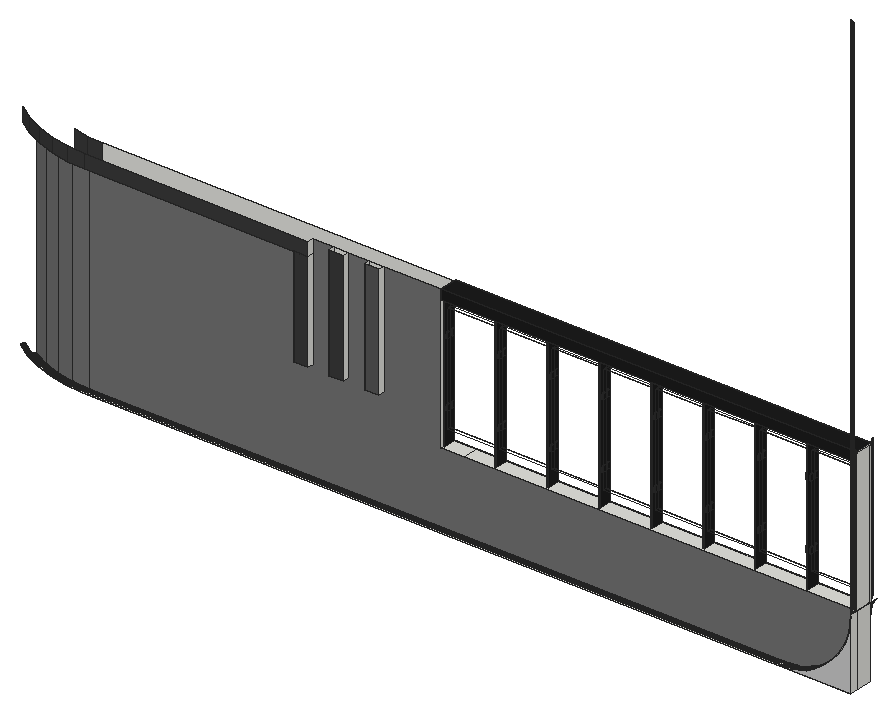
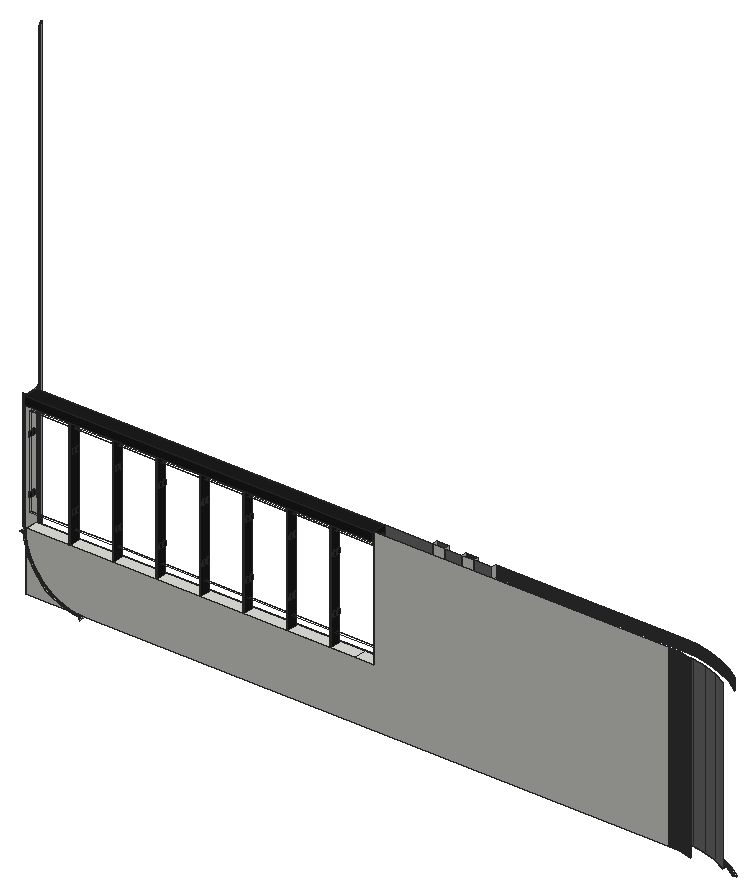
# SketchUp Ruby script. Lengths in inches.
U = 1.inch
M = Sketchup.active_model
def pt(a) = Geom::Point3d.new(a.map { |v| v * U })
def face(e, loops, mat)
  f = e.add_face(loops[0].map { |a| pt(a) })
  loops[1..].each { |l| e.add_face(l.map { |a| pt(a) }).erase! }
  f.material = f.back_material = mat if mat
  f
end
# faces: each face lists its corners as indices into pts; further lists are holes
def faces(e, pts, list, mat = nil) = list.each { |f| face(e, (f[0].is_a?(Array) ? f : [f]).map { |l| l.map { |i| pts[i] } }, mat) }
# xy, xz, yz: faces in a plane at the given z, y or x. An outline is a flat list of corners, or four numbers for a rectangle; further outlines are holes
def ring(l) = l.size == 4 ? [[l[0], l[1]], [l[2], l[1]], [l[2], l[3]], [l[0], l[3]]] : l.each_slice(2).to_a
def flat(e, list, mat, &to3) = list.each { |f| face(e, (f[0].is_a?(Array) ? f : [f]).map { |l| ring(l).map { |u, v| to3.(u, v) } }, mat) }
def xy(e, z, list, mat = nil) = flat(e, list, mat) { |x, y| [x, y, z] }
def xz(e, y, list, mat = nil) = flat(e, list, mat) { |x, z| [x, y, z] }
def yz(e, x, list, mat = nil) = flat(e, list, mat) { |y, z| [x, y, z] }
def lines(e, pts, list) = list.each { |a, b| e.add_line(pt(pts[a]), pt(pts[b])) }
# prism: a flat outline (further loops are holes) pulled along v
def prism(e, loops, v, mat = nil)
  f = face(e, loops, mat); d = Geom::Vector3d.new(v.map { |x| x * U })
  f.pushpull(f.normal.samedirection?(d) ? d.length : -d.length)
end
def box(e, o, s, mat = nil) = prism(e, [[o, [o[0] + s[0], o[1], o[2]], [o[0] + s[0], o[1] + s[1], o[2]], [o[0], o[1] + s[1], o[2]]]], [0, 0, s[2]], mat)
def at(x, y, z, deg = 0) = Geom::Transformation.translation(pt([x, y, z])) * Geom::Transformation.rotation(ORIGIN, Z_AXIS, deg.degrees)
def axes(o, x, y, z) = Geom::Transformation.new([*x, 0, *y, 0, *z, 0, *pt(o).to_a, 1])
def part(name) = M.definitions.add(name)
# library, detail: a bought-in or finely detailed component or shape, given as its bounding box
def library(name, o, s) = part(name).tap { |d| box(d.entities, o, s) }
def detail(e, o, s) = box(e.add_group.entities, o, s)
def put(e, d, t, mat = nil) = e.add_instance(d, t).tap { |i| i.material = mat if mat }
def group(e, t, mat = nil) = e.add_group.tap { |g| g.transformation = t; g.material = mat if mat }.entities
root = M.entities
M.materials.add("[0131_Silver]").color = [28, 28, 28]
M.materials.add("[Cladding Stucco White]").color = [200, 200, 200]
M.materials.add("[Color M05]").color = [114, 114, 114]
M.materials.add("[Color M06]").color = [86, 86, 86]
M.materials.add("[Color M07]").color = [58, 58, 58]
M.materials.add("[Translucent_Glass_Blue]").color = [255, 255, 255]
M.materials["[Translucent_Glass_Blue]"].alpha = 0
c1 = part("Group\#11")
xy(c1.entities,0,[[0,0,0.39,2.125]],"[0131_Silver]")
xy(c1.entities,1.5,[[0,0,0.39,2.125]],"[0131_Silver]")
xz(c1.entities,0,[[0,0,0.39,1.5]],"[0131_Silver]")
xz(c1.entities,2.125,[[0,0,0.39,1.5]],"[0131_Silver]")
yz(c1.entities,0,[[0,0,2.125,1.5]],"[0131_Silver]")
yz(c1.entities,0.39,[[0,0,2.125,1.5]],"[0131_Silver]")
c2 = part("Glass railing panel")
xy(c2.entities,0,[[-0.59,0,0,63.98]])
xy(c2.entities,37.71,[[-0.59,0,0,63.98]])
xz(c2.entities,0,[[-0.59,0,0,37.71]])
xz(c2.entities,63.98,[[-0.59,0,0,37.71]])
yz(c2.entities,-0.59,[[0,0,63.98,37.71]])
yz(c2.entities,0,[[0,0,63.98,0,63.98,37.71,0,37.71,0,30.53,1.75,30.53,1.75,28.71,0,28.71],[-0.4,28.71,0,30.53],[0,28.71,1.75,30.53]])
p = [[0,63.98,30.53],[0.39,63.98,30.53]]
lines(c2.entities,p,[[0,1]])
put(c2.entities,c1,axes([0,62.22,28.71],[1,0,0],[0,1.01246,0],[0,0,1.2158]))
put(c2.entities,c1,axes([0,62.22,6.27],[1,0,0],[0,1.01246,0],[0,0,1.2158]))
put(c2.entities,c1,axes([0,0.6,28.71],[1,0,0],[0,1.01246,0],[0,0,1.2158]))
put(c2.entities,c1,axes([0,0.6,6.27],[1,0,0],[0,1.01246,0],[0,0,1.2158]))
put(c2.entities,c1,axes([-0.98,0.6,28.71],[1,0,0],[0,1.01246,0],[0,0,1.2158]))
put(c2.entities,c1,axes([-0.98,62.22,6.27],[1,0,0],[0,1.01246,0],[0,0,1.2158]))
put(c2.entities,c1,axes([-0.98,0.6,6.27],[1,0,0],[0,1.01246,0],[0,0,1.2158]))
put(c2.entities,c1,axes([-0.98,62.22,28.71],[1,0,0],[0,1.01246,0],[0,0,1.2158]))
c3 = part("Group\#1")
xz(c3.entities,0,[[0,0,1.97,38.58]])
xz(c3.entities,1.97,[[0,0,1.97,38.58]])
yz(c3.entities,0,[[0,0,1.97,37.71]])
yz(c3.entities,1.97,[[0,0,1.97,37.71]])
c4 = part("Glass railing section")
xy(c4.entities,37.71,[[2.51,0,3.15,0.39,3.15,0]])
xy(c4.entities,37.71,[[0,0,0.54,520.67],[2.51,0,2.51,63.58,3.15,0.39],[3.15,0.39,2.51,63.58,2.51,520.67,3.15,520.67]],"[0131_Silver]")
xy(c4.entities,38.58,[[0.54,496.0625,2.51,520.67]])
xy(c4.entities,38.58,[[0.54,0,2.51,496.0625]],"[0131_Silver]")
xy(c4.entities,40.46,[[0,0,3.15,520.67]],"[0131_Silver]")
xz(c4.entities,0,[[0,37.71,0.54,37.71,0.54,38.58,2.51,38.58,2.51,37.71,3.15,37.71,3.15,40.46,0,40.46]],"[0131_Silver]")
xz(c4.entities,520.67,[[0,37.71,0,40.46,3.15,40.46,3.15,37.71,2.51,37.71,2.51,38.58,0.54,38.58,0.54,37.71]])
yz(c4.entities,0,[[0,37.71,520.67,40.46]],"[0131_Silver]")
yz(c4.entities,0.54,[[496.0625,37.71,520.67,38.58]])
yz(c4.entities,0.54,[[0,37.71,496.0625,38.58]],"[0131_Silver]")
yz(c4.entities,2.51,[[0,37.71,496.0625,38.58],[496.0625,37.71,520.67,38.58]])
yz(c4.entities,3.15,[[0,37.71,520.67,40.46]],"[0131_Silver]")
put(c4.entities,c2,axes([1.8,65.35,3.9375],[1,0,0],[0,0.98769,0],[0,0,0.8225]),"[Translucent_Glass_Blue]")
put(c4.entities,c2,axes([1.8,130.31,3.9375],[1,0,0],[0,0.98769,0],[0,0,0.8225]),"[Translucent_Glass_Blue]")
put(c4.entities,c2,axes([1.8,195.28,3.9375],[1,0,0],[0,0.98769,0],[0,0,0.8225]),"[Translucent_Glass_Blue]")
put(c4.entities,c2,axes([1.8,260.24,3.9375],[1,0,0],[0,0.98769,0],[0,0,0.8225]),"[Translucent_Glass_Blue]")
put(c4.entities,c2,axes([1.8,325.2,3.9375],[1,0,0],[0,0.98769,0],[0,0,0.8225]),"[Translucent_Glass_Blue]")
put(c4.entities,c2,axes([1.8,390.16,3.9375],[1,0,0],[0,0.98769,0],[0,0,0.8225]),"[Translucent_Glass_Blue]")
put(c4.entities,c2,axes([1.8,455.12,3.9375],[1,0,0],[0,0.98769,0],[0,0,0.8225]),"[Translucent_Glass_Blue]")
put(c4.entities,c2,axes([1.8,0.39,3.9375],[1,0,0],[0,0.98769,0],[0,0,0.8225]),"[Translucent_Glass_Blue]")
put(c4.entities,c3,at(0.54,128.9375,0),"[0131_Silver]")
g1 = group(c4.entities,at(0.54,63.98,0),"[0131_Silver]")
xz(g1,0,[[0,0,1.97,38.58]])
xz(g1,1.97,[[0,0,1.97,38.58]])
yz(g1,0,[[0,0,1.97,37.71]])
yz(g1,1.97,[[0,0,1.97,37.71]])
put(c4.entities,c3,at(0.54,193.9,0),"[0131_Silver]")
put(c4.entities,c3,at(0.54,258.86,0),"[0131_Silver]")
put(c4.entities,c3,at(0.54,323.82,0),"[0131_Silver]")
put(c4.entities,c3,at(0.54,388.78,0),"[0131_Silver]")
put(c4.entities,c3,at(0.54,453.74,0),"[0131_Silver]")
put(c4.entities,c3,at(0.54,518.7,0),"[0131_Silver]")
c5 = part("Glass+Railing")
put(c5.entities,c4,axes([0,0,0],[1,0,0],[0,0.95652,0],[0,0,1]),"[0131_Silver]")
xy(root,126,[[142.019,1,154.019,2.33],[142.019,2.33,154.019,5.061]])
xy(root,126.103,[[24.213,1.209,24.213,1.212,21.145,1.413,21.144,1.41],[24.213,1.209,24.257,1.209,24.213,1.212],[21.144,1.41,21.145,1.413,18.093,2.02,18.092,2.017],[18.092,2.017,18.093,2.02,15.146,3.02,15.145,3.018],[21.264,2.317,21.264,2.32,18.329,2.903,18.328,2.901],
  [18.328,2.901,18.329,2.903,15.496,3.865,15.495,3.863],[15.145,3.018,15.146,3.02,12.355,4.397,12.353,4.394],[15.495,3.863,15.496,3.865,12.812,5.189,12.811,5.186],[12.353,4.394,12.355,4.397,9.767,6.126,9.765,6.123]])
xy(root,126.14,[[24.217,1.32,24.217,1.322,21.159,1.523,21.159,1.52],[24.217,1.32,24.26,1.32,24.217,1.322],[21.159,1.52,21.159,1.523,18.121,2.127,18.121,2.124],[18.121,2.124,18.121,2.127,15.188,3.123,15.187,3.12],[21.249,2.207,21.25,2.21,18.301,2.796,18.3,2.793],
  [18.3,2.793,18.301,2.796,15.453,3.763,15.452,3.76],[15.187,3.12,15.188,3.123,12.41,4.493,12.409,4.49],[15.452,3.76,15.453,3.763,12.756,5.093,12.755,5.09],[12.409,4.49,12.41,4.493,9.835,6.214,9.833,6.211]])
xy(root,126.166,[[24.221,1.433,24.221,1.436,21.174,1.636,21.174,1.633],[24.221,1.433,24.264,1.433,24.221,1.436],[21.174,1.633,21.174,1.636,18.151,2.237,18.15,2.234],[24.236,1.897,24.236,1.9,21.235,2.097,21.234,2.094],[24.236,1.897,24.279,1.897,24.236,1.9],
  [21.234,2.094,21.235,2.097,18.271,2.686,18.27,2.684],[18.15,2.234,18.151,2.237,15.232,3.228,15.231,3.225],[18.27,2.684,18.271,2.686,15.41,3.658,15.409,3.655],[15.231,3.225,15.232,3.228,12.467,4.591,12.466,4.589],[15.409,3.655,15.41,3.658,12.7,4.994,12.698,4.992],
  [12.466,4.589,12.467,4.591,9.904,6.304,9.902,6.302]])
xy(root,126.182,[[24.224,1.549,24.225,1.552,21.189,1.751,21.189,1.748],[24.224,1.549,24.268,1.549,24.225,1.552],[21.189,1.748,21.189,1.751,18.181,2.349,18.18,2.346],[24.232,1.782,24.232,1.785,21.22,1.982,21.219,1.979],[24.232,1.782,24.276,1.782,24.232,1.785],
  [21.219,1.979,21.22,1.982,18.241,2.574,18.24,2.572],[18.18,2.346,18.181,2.349,15.276,3.335,15.275,3.332],[18.24,2.572,18.241,2.574,15.365,3.551,15.364,3.548],[15.275,3.332,15.276,3.335,12.525,4.692,12.524,4.689],[15.364,3.548,15.365,3.551,12.642,4.894,12.64,4.891],
  [12.524,4.689,12.525,4.692,9.974,6.396,9.973,6.394]])
xy(root,126.1875,[[24.228,1.665,24.228,1.668,21.204,1.866,21.204,1.863],[24.228,1.665,24.272,1.665,24.228,1.668],[21.204,1.863,21.204,1.866,18.211,2.462,18.211,2.46,18.21,2.459],[18.21,2.459,18.211,2.46,18.211,2.462,15.321,3.443,15.32,3.441,15.32,3.44],[15.32,3.44,15.32,3.441,15.321,3.443,12.583,4.793,12.583,4.791,12.582,4.79],
  [12.582,4.79,12.583,4.791,12.583,4.793,10.046,6.488,10.044,6.486]])
xy(root,137.896,[[83.599,2.33,87.474,5.061],[87.474,2.33,153.974,5.061]])
xy(root,142.9375,[[59.529,1.33,61.967,2.33],[65.529,1.33,67.967,2.33],[71.529,1.33,73.967,2.33]])
xz(root,1,[[142.019,126,154.019,126,154.019,138,153.916,136.434,153.61,134.894,153.105,133.408,152.411,132,151.539,130.695,150.504,129.515,149.324,128.48,148.019,127.608,146.611,126.913,145.124,126.409,143.585,126.103]],"[Cladding Stucco White]")
xz(root,1.33,[[71.529,142.9375,73.967,162]],"[Color M06]")
xz(root,1.33,[[59.529,142.9375,61.967,159.6875],[65.529,142.9375,67.967,162],[24.217,159.6875,61.967,162]],"[Color M07]")
xz(root,2.33,[[65.529,142.9375,67.967,162],[71.529,142.9375,73.967,162]])
xz(root,2.33,[[24.25,126,154.019,126,154.019,162,153.974,137.896,83.599,137.896,83.599,162,73.967,162,73.967,142.9375,71.529,142.9375,71.529,162,67.967,162,67.967,142.9375,65.529,142.9375,65.529,162,61.967,162,61.967,142.9375,59.529,142.9375,59.529,159.6875,24.25,159.6875]],"[Color M05]")
xz(root,5.061,[[24.25,126,24.25,162,83.599,162,83.599,137.896,153.974,137.896,154.019,162,154.019,126]])
yz(root,59.529,[[1.33,142.9375,2.33,159.6875]])
yz(root,61.967,[[1.33,142.9375,2.33,159.6875],[1.33,159.6875,2.33,162]])
yz(root,65.529,[[1.33,142.9375,2.33,162]])
yz(root,67.967,[[1.33,142.9375,2.33,162]])
yz(root,71.529,[[1.33,142.9375,2.33,162]])
yz(root,73.967,[[1.33,142.9375,2.33,162]])
yz(root,83.599,[[2.33,137.896,5.061,162]])
yz(root,154.019,[[1,126,2.33,138],[2.33,126,5.061,138],[2.33,138,5.061,162]])
p = [[24.25,1,126],[24.253,1.102,126.056],[21.131,1.307,126.056],[21.117,1.205,126],[24.207,1.003,126],[21.13,1.304,126.056],
  [21.117,1.202,126],[24.206,1,126],[24.21,1.102,126.056],[140.688,1,126],[142.019,1,126],[141.916,1.102,126.056],
  [140.79,1.102,126.056],[142.019,2.33,126],[141.916,2.228,126.056],[142.123,1.107,126.045],[143.585,1,126.103],[143.58,1.107,126.14],
  [142.123,2.33,126.045],[142.123,5.061,126.045],[142.123,6.284,126.045],[142.019,6.391,126],[142.019,5.061,126],[142.23,1.216,126.083],
  [143.576,1.216,126.171],[142.23,2.33,126.083],[142.23,5.061,126.083],[142.23,6.175,126.083],[18.064,1.914,126.056],[18.038,1.815,126],
  [18.065,1.917,126.056],[18.038,1.818,126],[15.104,2.919,126.056],[15.065,2.824,126],[15.105,2.921,126.056],[15.066,2.827,126],
  [21.291,2.524,126],[21.278,2.423,126.056],[24.247,2.228,126.056],[24.25,2.33,126],[24.29,2.228,126.056],[24.294,2.33,126],
  [21.291,2.527,126],[21.291,2.524,126.002],[21.278,2.426,126.056],[140.688,2.33,126],[140.79,2.228,126.056],[24.25,2.33,159.6875],
  [21.291,2.524,159.6875],[18.383,3.103,126],[18.356,3.004,126.056],[18.383,3.106,126],[18.383,3.103,126.002],[18.357,3.007,126.056],
  [18.383,3.103,159.6875],[12.3,4.302,126.056],[12.249,4.213,126],[12.301,4.304,126.056],[12.25,4.215,126],[15.575,4.056,126],
  [15.536,3.961,126.056],[15.576,4.059,126],[15.575,4.056,126.002],[15.537,3.964,126.056],[15.575,4.056,159.6875],[12.915,5.368,126],
  [12.864,5.279,126.056],[12.917,5.37,126],[12.915,5.368,126.002],[12.865,5.281,126.056],[12.915,5.368,159.6875],[9.7,6.038,126.056],
  [9.638,5.957,126],[9.702,6.041,126.056],[9.64,5.96,126],[24.25,5.061,126],[21.647,5.231,126],[21.647,5.231,162],
  [24.25,5.061,162],[19.089,5.74,126],[19.089,5.74,162],[145.124,1,126.409],[145.115,1.107,126.445],[24.257,1.209,126.103],
  [24.213,1.212,126.103],[21.145,1.413,126.103],[21.144,1.41,126.103],[24.213,1.209,126.103],[141.81,1.209,126.103],[140.897,1.209,126.103],
  [141.81,2.121,126.103],[145.106,1.216,126.476],[24.26,1.32,126.14],[24.217,1.322,126.14],[21.159,1.523,126.14],[21.159,1.52,126.14],
  [24.217,1.32,126.14],[141.699,1.32,126.14],[141.008,1.32,126.14],[141.699,2.011,126.14],[142.339,1.327,126.114],[143.573,1.327,126.195],
  [142.339,6.064,126.114],[142.339,2.33,126.114],[142.339,5.061,126.114],[18.092,2.017,126.103],[18.093,2.02,126.103],[24.264,1.433,126.166],
  [24.221,1.436,126.166],[21.174,1.636,126.166],[21.174,1.633,126.166],[24.221,1.433,126.166],[141.585,1.433,126.166],[141.121,1.433,126.166],
  [141.585,1.897,126.166],[142.449,1.439,126.139],[143.57,1.439,126.213],[142.449,5.952,126.139],[142.449,2.33,126.139],[142.449,5.061,126.139],
  [18.121,2.124,126.14],[142.561,1.552,126.157],[143.569,1.552,126.223],[142.561,2.33,126.157],[142.561,5.061,126.157],[142.561,5.839,126.157],
  [18.15,2.234,126.166],[18.121,2.127,126.14],[15.145,3.018,126.103],[15.146,3.02,126.103],[24.279,1.897,126.166],[24.283,2.011,126.14],
  [24.24,2.013,126.139],[21.25,2.21,126.14],[21.249,2.207,126.14],[21.235,2.097,126.166],[24.236,1.9,126.166],[24.24,2.011,126.14],
  [141.121,1.897,126.166],[141.008,2.011,126.14],[15.187,3.12,126.14],[24.287,2.121,126.103],[21.264,2.32,126.103],[21.264,2.317,126.103],
  [24.243,2.121,126.103],[140.897,2.121,126.103],[143.126,2.114,126.142],[143.014,2.004,126.159],[143.573,2.004,126.195],[143.576,2.114,126.171],
  [143.126,5.277,126.142],[143.014,5.388,126.159],[143.014,5.061,126.159],[143.014,2.33,126.159],[143.126,2.33,126.142],[143.126,5.061,126.142],
  [15.231,3.225,126.166],[15.188,3.123,126.14],[18.3,2.793,126.14],[18.271,2.686,126.166],[143.237,2.223,126.118],[143.58,2.223,126.14],
  [143.237,5.168,126.118],[143.237,2.33,126.118],[143.237,5.061,126.118],[145.106,2.114,126.476],[145.115,2.223,126.445],[18.328,2.901,126.103],
  [18.301,2.796,126.14],[143.346,2.33,126.087],[143.585,2.33,126.103],[143.346,5.061,126.087],[145.124,2.33,126.409],[18.329,2.903,126.103],
  [143.585,5.061,126.103],[145.124,5.061,126.409],[15.452,3.76,126.14],[15.41,3.658,126.166],[15.495,3.863,126.103],[15.453,3.763,126.14],
  [12.353,4.394,126.103],[12.355,4.397,126.103],[15.496,3.865,126.103],[12.409,4.49,126.14],[12.466,4.589,126.166],[12.41,4.493,126.14],
  [12.755,5.09,126.14],[12.7,4.994,126.166],[12.811,5.186,126.103],[12.756,5.093,126.14],[12.812,5.189,126.103],[9.765,6.123,126.103],
  [9.767,6.126,126.103],[9.833,6.211,126.14],[9.902,6.302,126.166],[9.835,6.214,126.14],[143.58,5.168,126.14],[145.115,5.168,126.445],
  [143.576,5.277,126.171],[145.106,5.277,126.476],[143.573,5.388,126.195],[145.1,1.327,126.499],[145.096,1.439,126.516],[24.268,1.549,126.182],
  [24.225,1.552,126.182],[21.189,1.751,126.182],[21.189,1.748,126.182],[24.224,1.549,126.182],[141.47,1.549,126.182],[141.237,1.549,126.182],
  [141.47,1.782,126.182],[145.093,1.552,126.526],[24.272,1.665,126.1875],[24.228,1.668,126.1875],[21.204,1.866,126.1875],[21.204,1.865,126.1875],
  [21.204,1.863,126.1875],[24.228,1.665,126.1875],[141.353,1.665,126.1875],[18.18,2.346,126.182],[18.151,2.237,126.166],[142.674,1.665,126.168],
  [143.569,1.665,126.227],[142.674,2.33,126.168],[142.674,5.061,126.168],[142.674,5.726,126.168],[145.092,1.665,126.53],[21.22,1.982,126.182],
  [21.219,1.979,126.182],[24.232,1.782,126.182],[24.276,1.782,126.182],[24.232,1.785,126.182],[141.237,1.782,126.182],[142.788,1.779,126.172],
  [143.569,1.779,126.223],[142.788,2.33,126.172],[142.788,5.061,126.172],[142.788,5.613,126.172],[145.093,1.779,126.526],[18.21,2.459,126.1875],
  [18.181,2.349,126.182],[21.234,2.094,126.166],[24.236,1.897,126.166],[142.901,1.892,126.169],[143.57,1.892,126.213],[142.901,2.33,126.169],
  [142.901,5.061,126.169],[142.901,5.5,126.169],[145.096,1.892,126.516],[18.24,2.572,126.182],[18.211,2.462,126.1875],[145.1,2.004,126.499],
  [18.27,2.684,126.166],[18.241,2.574,126.182],[15.275,3.332,126.182],[15.232,3.228,126.166],[15.32,3.44,126.1875],[15.276,3.335,126.182],
  [15.364,3.548,126.182],[15.321,3.443,126.1875],[15.409,3.655,126.166],[15.365,3.551,126.182],[12.524,4.689,126.182],[12.467,4.591,126.166],
  [12.582,4.79,126.1875],[12.525,4.692,126.182],[12.64,4.891,126.182],[12.583,4.793,126.1875],[12.698,4.992,126.166],[12.642,4.894,126.182],
  [9.973,6.394,126.182],[9.904,6.304,126.166],[10.044,6.486,126.1875],[9.974,6.396,126.182],[145.1,5.388,126.499],[143.57,5.5,126.213],
  [145.096,5.5,126.516],[143.569,5.613,126.223],[145.093,5.613,126.526],[143.569,5.726,126.227],[145.092,5.726,126.53],[146.611,1,126.913],
  [146.596,1.107,126.948],[146.584,1.216,126.977],[146.584,2.114,126.977],[146.596,2.223,126.948],[146.611,2.33,126.913],[146.611,5.061,126.913],
  [146.596,5.168,126.948],[146.584,5.277,126.977],[146.575,1.327,127],[146.568,1.439,127.016],[146.564,1.552,127.026],[146.563,1.665,127.029],
  [146.564,1.779,127.026],[146.568,1.892,127.016],[146.575,2.004,127],[146.575,5.388,127],[146.568,5.5,127.016],[146.564,5.613,127.026],
  [146.563,5.726,127.029],[148.019,1,127.608],[148,1.107,127.641],[147.984,1.216,127.668],[147.984,2.114,127.668],[148,2.223,127.641],
  [148.019,2.33,127.608],[148.019,5.061,127.608],[148,5.168,127.641],[147.984,5.277,127.668],[147.972,1.327,127.689],[147.963,1.439,127.704],
  [147.958,1.552,127.713],[147.956,1.665,127.716],[147.958,1.779,127.713],[147.963,1.892,127.704],[147.972,2.004,127.689],[147.972,5.388,127.689],
  [147.963,5.5,127.704],[147.958,5.613,127.713],[147.956,5.726,127.716],[149.324,1,128.48],[149.301,1.107,128.51],[149.282,1.216,128.535],
  [149.282,2.114,128.535],[149.301,2.223,128.51],[149.324,2.33,128.48],[149.324,5.061,128.48],[149.301,5.168,128.51],[149.282,5.277,128.535],
  [149.267,1.327,128.554],[149.256,1.439,128.568],[149.25,1.552,128.576],[149.248,1.665,128.579],[149.25,1.779,128.576],[149.256,1.892,128.568],
  [149.267,2.004,128.554],[149.267,5.388,128.554],[149.256,5.5,128.568],[149.25,5.613,128.576],[149.248,5.726,128.579],[150.504,1,129.515],
  [150.477,1.107,129.542],[150.455,1.216,129.564],[150.438,1.327,129.581],[150.438,2.004,129.581],[150.455,2.114,129.564],[150.477,2.223,129.542],
  [150.504,2.33,129.515],[150.504,5.061,129.515],[150.477,5.168,129.542],[150.455,5.277,129.564],[150.438,5.388,129.581],[150.425,1.439,129.593],
  [150.418,1.552,129.601],[150.415,1.665,129.603],[150.418,1.779,129.601],[150.425,1.892,129.593],[150.425,5.5,129.593],[150.418,5.613,129.601],
  [150.415,5.726,129.603],[151.539,1,130.695],[151.509,1.107,130.718],[151.484,1.216,130.737],[151.484,2.114,130.737],[151.509,2.223,130.718],
  [151.539,2.33,130.695],[151.539,5.061,130.695],[151.509,5.168,130.718],[151.484,5.277,130.737],[151.465,1.327,130.752],[151.451,1.439,130.762],
  [151.442,1.552,130.769],[151.44,1.665,130.771],[151.442,1.779,130.769],[151.451,1.892,130.762],[151.465,2.004,130.752],[151.465,5.388,130.752],
  [151.451,5.5,130.762],[151.442,5.613,130.769],[152.411,1,132],[152.378,1.107,132.019],[152.351,1.216,132.035],[152.33,1.327,132.047],
  [152.33,2.004,132.047],[152.351,2.114,132.035],[152.378,2.223,132.019],[152.411,2.33,132],[152.411,5.061,132],[152.378,5.168,132.019],
  [152.351,5.277,132.035],[152.33,5.388,132.047],[152.315,1.439,132.055],[152.306,1.552,132.061],[152.303,1.665,132.0625],[152.306,1.779,132.061],
  [152.315,1.892,132.055],[152.315,5.5,132.055],[152.306,5.613,132.061],[153.105,1,133.408],[153.07,1.107,133.422],[153.041,1.216,133.434],
  [153.019,1.327,133.444],[153.003,1.439,133.45],[153.003,1.892,133.45],[153.019,2.004,133.444],[153.041,2.114,133.434],[153.07,2.223,133.422],
  [153.105,2.33,133.408],[153.105,5.061,133.408],[153.07,5.168,133.422],[153.041,5.277,133.434],[153.019,5.388,133.444],[153.003,5.5,133.45],
  [152.993,1.552,133.454],[152.99,1.665,133.456],[152.993,1.779,133.454],[152.993,5.613,133.454],[153.61,1,134.894],[153.573,1.107,134.904],
  [153.543,1.216,134.912],[153.519,1.327,134.918],[153.502,1.439,134.923],[153.502,1.892,134.923],[153.519,2.004,134.918],[153.543,2.114,134.912],
  [153.573,2.223,134.904],[153.61,2.33,134.894],[153.61,5.061,134.894],[153.573,5.168,134.904],[153.543,5.277,134.912],[153.519,5.388,134.918],
  [153.502,5.5,134.923],[153.492,1.552,134.926],[153.489,1.665,134.927],[153.492,1.779,134.926],[153.492,5.613,134.926],[153.916,1,136.434],
  [153.878,1.107,136.439],[153.847,1.216,136.443],[153.823,1.327,136.446],[153.806,1.439,136.448],[153.795,1.552,136.45],[153.792,1.665,136.45],
  [153.795,1.779,136.45],[153.806,1.892,136.448],[153.823,2.004,136.446],[153.847,2.114,136.443],[153.878,2.223,136.439],[153.916,2.33,136.434],
  [153.916,5.061,136.434],[153.878,5.168,136.439],[153.847,5.277,136.443],[153.823,5.388,136.446],[153.806,5.5,136.448],[153.795,5.613,136.45],
  [154.019,1,138],[153.974,1.107,137.896],[153.936,1.216,137.789],[153.904,1.327,137.68],[153.879,1.439,137.569],[153.861,1.552,137.457],
  [153.851,1.665,137.344],[153.847,1.779,137.231],[153.85,1.892,137.118],[153.86,2.004,137.005],[153.877,2.114,136.892],[153.901,2.223,136.782],
  [153.932,2.33,136.672],[153.932,5.061,136.672],[153.901,5.168,136.782],[153.877,5.277,136.892],[153.86,5.388,137.005],[153.85,5.5,137.118],
  [153.847,5.613,137.231],[153.901,2.33,136.782],[153.901,5.061,136.782],[153.877,2.33,136.892],[153.877,5.061,136.892],[153.86,5.061,137.005],
  [153.86,2.33,137.005],[153.85,2.33,137.118],[153.85,5.061,137.118],[153.847,5.061,137.231],[153.847,2.33,137.231],[153.851,5.061,137.344],
  [153.851,5.726,137.344],[153.851,2.33,137.344],[153.861,2.33,137.457],[153.861,5.061,137.457],[153.861,5.839,137.457],[153.879,2.33,137.569],
  [153.879,5.061,137.569],[153.879,5.952,137.569],[153.904,5.061,137.68],[153.904,6.064,137.68],[153.904,2.33,137.68],[153.936,5.061,137.789],
  [153.936,6.175,137.789],[153.936,2.33,137.789],[153.974,5.061,137.896],[153.974,6.284,137.896],[153.974,2.33,137.896],[154.019,5.061,138],
  [154.019,6.391,138],[154.019,2.33,138],[154.019,2.33,162],[154.019,5.061,162],[154.001,1.11,163.221],[154.001,1.11,139.221],
  [154.001,1.11,138.11],[154.019,1,139.33],[154.019,1,163.33],[154.019,1,228],[154.001,1.11,227.89],[154.001,2.221,138.11],
  [154.001,2.221,139.221],[154.001,2.221,162.11],[154.019,2.33,139.33],[154.019,5.061,139.33],[154.001,5.171,162.11],[154.001,5.171,139.221],
  [154.001,5.171,138.11],[153.987,1.22,138.22],[153.987,1.22,227.78],[153.987,1.22,163.11],[153.987,1.22,139.11],[153.987,2.11,138.22],
  [153.987,2.11,139.11],[153.987,2.11,162.22],[153.987,5.281,162.22],[153.987,5.281,139.11],[153.987,5.281,138.22],[153.975,1.331,138.331],
  [153.975,1.331,227.669],[153.975,1.331,162.999],[153.975,1.331,138.999],[153.975,1.999,138.331],[153.975,1.999,138.999],[153.975,1.999,162.331],
  [153.975,5.392,162.331],[153.975,5.392,138.999],[153.975,5.392,138.331],[153.967,1.442,138.442],[153.967,1.442,227.558],[153.967,1.442,162.888],
  [153.967,1.442,138.888],[153.967,1.888,138.442],[153.967,1.888,138.888],[153.967,1.888,162.442],[153.967,5.503,162.442],[153.967,5.503,138.888],
  [153.967,5.503,138.442],[153.963,1.554,138.554],[153.963,1.554,227.446],[153.963,1.554,162.777],[153.963,1.554,138.777],[153.963,1.777,138.554],
  [153.963,1.777,138.777],[153.963,1.777,162.554],[153.963,5.615,162.554],[153.963,5.615,138.777],[153.963,5.615,138.554],[153.961,1.665,162.665],
  [153.961,1.665,138.665],[153.961,1.665,227.335],[153.961,5.726,162.665],[153.961,5.726,138.665],[21.16,1.531,162],[21.16,1.531,159.6875],
  [24.217,1.33,159.6875],[24.217,1.33,162],[18.123,2.135,162],[18.123,2.135,159.6875],[15.191,3.13,162],[15.191,3.13,159.6875],
  [12.414,4.5,162],[12.414,4.5,159.6875],[9.84,6.22,162],[9.84,6.22,159.6875]]
faces(root,p,[[0,1,2,3,4],[5,6,7,8],[8,7,0,9,10,11,12,1],[13,14,11,10],[13,10,15,18,19,20,21,22],[18,15,23,25,26,27,20,19],[28,29,6,5],[3,2,30,31],
  [32,33,29,28],[31,30,34,35],[36,37,38,39],[40,41,42,43,44],[38,40,41,39],[45,41,40,46,14,13],[49,50,37,36],[43,42,51,52,53,44],
  [55,56,33,32],[35,34,57,58],[59,60,50,49],[52,51,61,62,63,53],[65,66,60,59],[62,61,67,68,69,63],[71,72,56,55],[58,57,73,74],
  [1,83,84,85,2],[86,5,8,87],[11,88,89,83,87,8,1,12],[14,90,88,11],[83,92,93,94,95,85,84],[95,85,84,96],[96,84,83,89,88,97,98,92],[90,99,97,88],
  [102,27,26,25,23,100,103,104],[105,28,5,86],[2,85,106,30],[92,107,108,109,110,94,93],[110,94,93,111],[111,93,92,98,97,112,113,107],[99,114,112,97],[117,102,104,103,100,115,118,119],
  [120,106,85,95],[118,115,121,123,124,125,117,119],[126,127,94,110],[128,32,28,105],[30,106,129,34],[130,131,132,133,134,135,136],[134,135,136,137],[137,136,130,138,114,99,139,131],
  [140,129,106,120],[137,132,133,134],[131,141,142,143,133,132],[143,133,132,144],[137,131,132],[144,132,131,139,99,90,145,141],[150,151,152,153,147,146,154,155],[156,157,127,126],
  [158,159,135,134],[37,143,144,38],[141,40,44,142],[38,144,141,145,90,14,46,40],[162,150,155,154,146,160,163,164],[167,168,133,143],[171,162,164,163,160,169],[50,167,143,37],
  [142,44,53,173],[170,174,171,169],[172,175,174,170],[176,177,159,158],[178,179,168,167],[180,55,32,128],[34,129,181,57],[60,178,167,50],
  [173,53,63,182],[183,181,129,140],[184,185,157,156],[186,187,177,176],[188,189,179,178],[66,188,178,60],[182,63,69,190],[191,71,55,180],
  [57,181,192,73],[193,192,181,183],[194,195,185,184],[174,196,162,171],[175,197,196,174],[196,198,150,162],[197,199,198,196],[198,200,151,150],
  [107,203,204,205,206,109,108],[206,109,108,207],[207,108,107,113,112,208,209,203],[114,210,208,112],[203,212,213,214,215,216,205,204],[217,204,203,209,208,218,212],[210,218,208],[219,220,109,206],
  [216,205,204,217],[123,121,221,223,224,225,125,124],[227,228,229,213,212,230,231],[214,213,229,228],[229,213,212,218,210,232,230],[223,221,233,235,236,237,225,224],[239,240,205,216],[230,130,136,135,241,227,231],
  [241,227,231,242],[242,231,230,232,210,114,138,130],[235,233,243,245,246,247,237,236],[249,250,214,228],[151,247,246,245,243,147,153,152],[252,253,227,241],[254,255,220,219],[256,257,240,239],
  [258,259,250,249],[260,261,253,252],[262,263,255,254],[264,265,257,256],[266,267,259,258],[268,269,261,260],[270,271,263,262],[272,273,265,264],
  [199,274,200,198],[200,275,247,151],[274,276,275,200],[275,277,237,247],[276,278,277,275],[277,279,225,237],[278,280,279,277],[286,287,175,172],
  [287,288,197,175],[288,289,199,197],[289,297,274,199],[297,298,276,274],[298,299,278,276],[299,300,280,278],[306,307,287,286],[307,308,288,287],
  [308,309,289,288],[309,317,297,289],[317,318,298,297],[318,319,299,298],[319,320,300,299],[326,327,307,306],[327,328,308,307],[328,329,309,308],
  [329,337,317,309],[337,338,318,317],[338,339,319,318],[339,340,320,319],[348,349,327,326],[349,350,328,327],[350,351,329,328],[351,352,337,329],
  [352,358,338,337],[358,359,339,338],[359,360,340,339],[366,367,349,348],[367,368,350,349],[368,369,351,350],[369,377,352,351],[377,378,358,352],
  [378,379,359,358],[387,388,367,366],[388,389,368,367],[389,390,369,368],[390,391,377,369],[391,397,378,377],[397,398,379,378],[408,409,388,387],
  [409,410,389,388],[410,411,390,389],[411,412,391,390],[412,413,397,391],[413,417,398,397],[427,428,409,408],[428,429,410,409],[429,430,411,410],
  [430,431,412,411],[431,432,413,412],[432,436,417,413],[449,450,428,427],[450,451,429,428],[451,452,430,429],[452,453,431,430],[453,454,432,431],
  [454,455,436,432],[450,449,468,469],[469,470,451,450],[470,471,452,451],[471,472,453,452],[472,473,454,453],[473,474,455,454],[468,467,475,476,470,469],
  [467,466,477,478,471,470,476,475],[479,472,471,478,477,466,465,480],[465,464,481,482,473,472,479,480],[483,474,473,482,481,464,463,484],[485,486,474,483,484,463,462,487],[462,461,488,489,490,486,485,487],[461,460,491,492,493,490,489,488],[494,495,493,492,491,460,459,496],
  [497,498,495,494,496,459,458,499],[500,501,498,497,499,458,457,502],[503,504,501,500,502,457,456,505],[502,506,507,500],[515,505,456,510],[519,507,520,521,522,503],[527,515,510,523],[521,520,530,531,532,522],
  [537,527,523,533],[531,530,540,541,542,532],[547,537,533,543],[541,540,550,551,552,542],[557,547,543,553],[551,550,560,561,562,552],[564,557,553],[561,560,566,567,562]])
faces(root,p,[[15,10,16,17],[23,15,17,24],[17,16,81,82],[24,17,82,91],[100,23,24,101],[115,100,101,116],[121,115,116,122],[146,147,148,149],
  [160,146,149,161],[161,149,165,166],[169,160,161,170],[170,161,166,172],[101,24,91,201],[116,101,201,202],[122,116,202,211],[221,121,122,222],
  [222,122,211,226],[233,221,222,234],[234,222,226,238],[243,233,234,244],[244,234,238,248],[147,243,244,148],[148,244,248,251],[149,148,251,165],
  [82,81,281,282],[91,82,282,283],[166,165,284,285],[172,166,285,286],[201,91,283,290],[202,201,290,291],[211,202,291,292],[226,211,292,293],
  [238,226,293,294],[248,238,294,295],[251,248,295,296],[165,251,296,284],[282,281,301,302],[283,282,302,303],[285,284,304,305],[286,285,305,306],
  [290,283,303,310],[291,290,310,311],[292,291,311,312],[293,292,312,313],[294,293,313,314],[295,294,314,315],[296,295,315,316],[284,296,316,304],
  [302,301,321,322],[303,302,322,323],[305,304,324,325],[306,305,325,326],[310,303,323,330],[311,310,330,331],[312,311,331,332],[313,312,332,333],
  [314,313,333,334],[315,314,334,335],[316,315,335,336],[304,316,336,324],[322,321,341,342],[323,322,342,343],[330,323,343,344],[324,336,345,346],
  [325,324,346,347],[326,325,347,348],[331,330,344,353],[332,331,353,354],[333,332,354,355],[334,333,355,356],[335,334,356,357],[336,335,357,345],
  [342,341,361,362],[343,342,362,363],[347,346,364,365],[348,347,365,366],[344,343,363,370],[353,344,370,371],[354,353,371,372],[355,354,372,373],
  [356,355,373,374],[357,356,374,375],[345,357,375,376],[346,345,376,364],[362,361,380,381],[363,362,381,382],[370,363,382,383],[364,376,384,385],
  [365,364,385,386],[366,365,386,387],[371,370,383,392],[372,371,392,393],[373,372,393,394],[374,373,394,395],[375,374,395,396],[376,375,396,384],
  [381,380,399,400],[382,381,400,401],[383,382,401,402],[392,383,402,403],[384,396,404,405],[385,384,405,406],[386,385,406,407],[387,386,407,408],
  [393,392,403,414],[394,393,414,415],[395,394,415,416],[396,395,416,404],[400,399,418,419],[401,400,419,420],[402,401,420,421],[403,402,421,422],
  [405,404,423,424],[406,405,424,425],[407,406,425,426],[408,407,426,427],[414,403,422,433],[415,414,433,434],[416,415,434,435],[404,416,435,423],
  [419,418,437,438],[420,419,438,439],[421,420,439,440],[422,421,440,441],[433,422,441,442],[434,433,442,443],[435,434,443,444],[423,435,444,445],
  [424,423,445,446],[425,424,446,447],[426,425,447,448],[427,426,448,449],[438,437,456,457],[439,438,457,458],[440,439,458,459],[441,440,459,460],
  [442,441,460,461],[443,442,461,462],[444,443,462,463],[445,444,463,464],[446,445,464,465],[447,446,465,466],[448,447,466,467],[449,448,467,468],
  [508,509,510,456,511,512,513,514],[516,517,506,518,505,515],[523,510,509,508,514,524,525,526],[528,529,517,516,515,527],[533,523,526,525,524,534,535,536],[538,539,529,528,527,537],[543,533,536,535,534,544,545,546],[548,549,539,538,537,547],
  [553,543,546,545,544,554,555,556],[558,559,549,548,547,557],[563,564,553,556,555,554,565],[564,563,559,558,557]],"[Cladding Stucco White]")
faces(root,p,[[36,39,47,48,43],[49,36,43,48,54,52],[59,49,52,54,64,62],[65,59,62,64,70,68]],"[Color M05]")
faces(root,p,[[75,76,77,78],[76,79,80,77],[568,569,570,571],[572,573,569,568],[574,575,573,572],[576,577,575,574],[578,579,577,576]],"[Color M07]")
put(root,c5,axes([153.97,2.33,137.9],[0,1,0],[-0.14131,0,0],[0,0,0.59571]))
